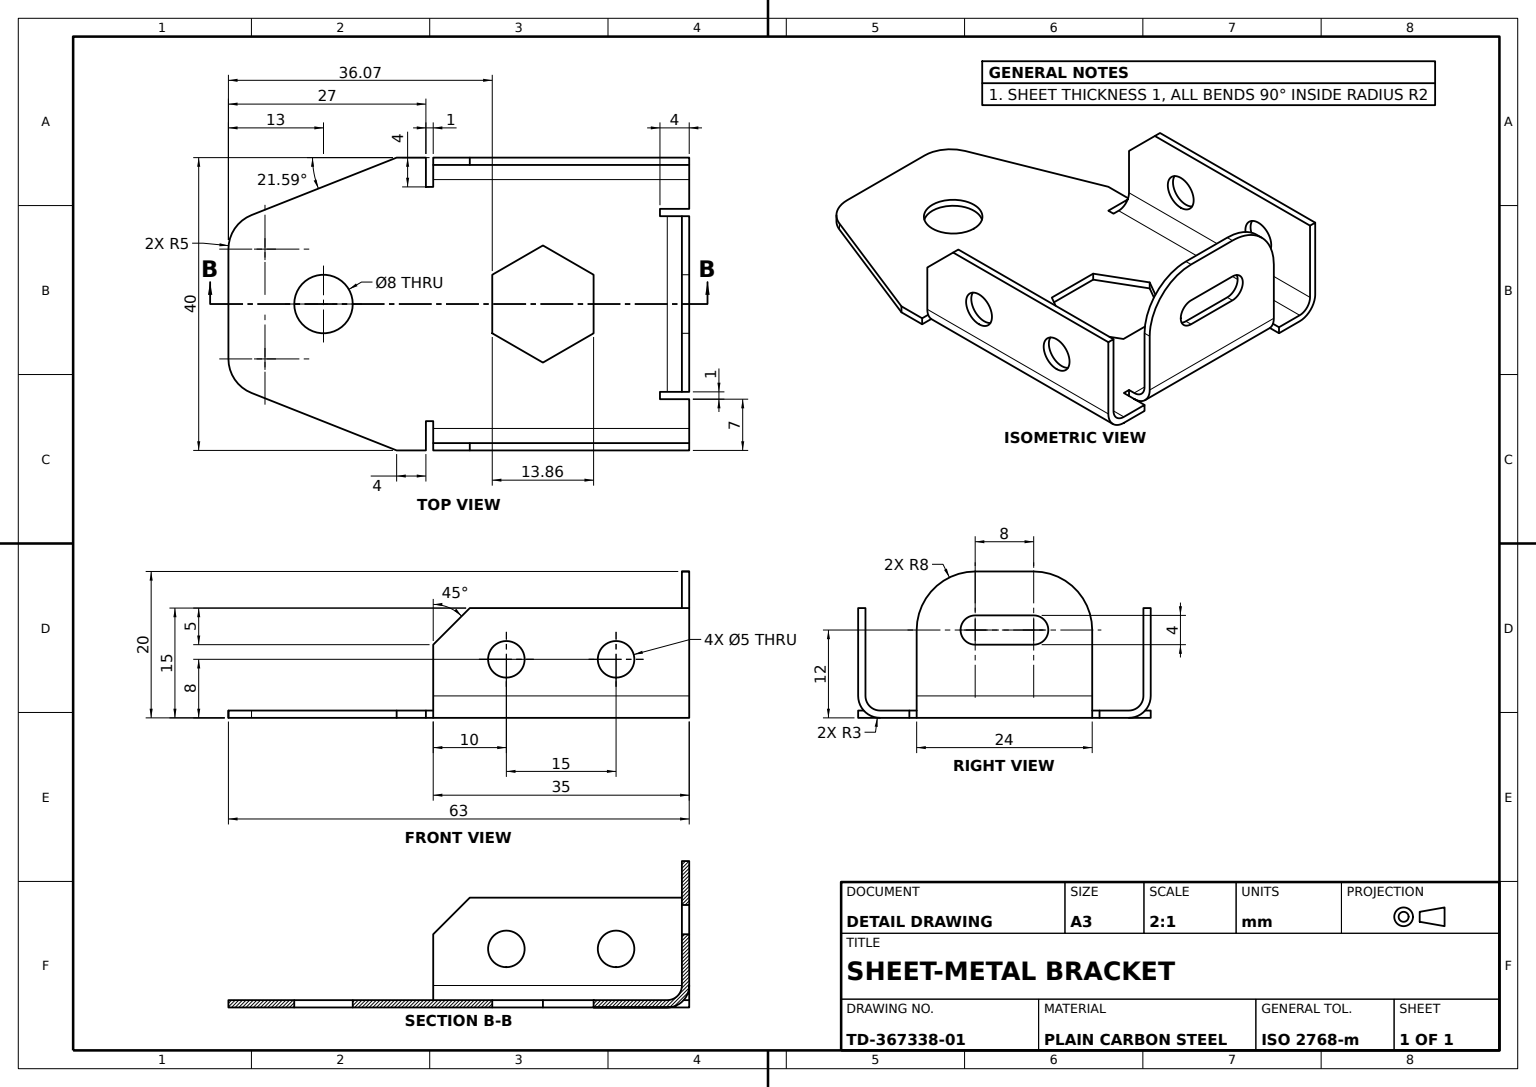
solid
v1 (20,9.5,-10)
v2 (20,4.5,-10)
e1 v1 v2 CIRCLE(AX(P(20,7,-10),D(1,0,0),D(0,1,0)),2.5)
e2 v2 v1 CIRCLE(AX(P(20,7,-10),D(1,0,0),D(0,1,0)),2.5)
v3 (20,2,-20)
v4 (20,2,15)
e3 v3 v4 LINE
v5 (20,14,-20)
e4 v3 v5 LINE
v6 (20,14,10)
e5 v5 v6 LINE
v7 (20,9,15)
e6 v6 v7 LINE
e7 v7 v4 LINE
v8 (20,9.5,5)
v9 (20,4.5,5)
e8 v8 v9 CIRCLE(AX(P(20,7,5),D(1,0,0),D(0,1,0)),2.5)
e9 v9 v8 CIRCLE(AX(P(20,7,5),D(1,0,0),D(0,1,0)),2.5)
face PLANE(AX(P(20,0,0),D(-1,0,0),D(0,-1,0))) rev [-e1 -e2] [-e3 e4 e5 e6 e7] [-e8 -e9]
v10 (-20,14,10)
v11 (-19,14,10)
e10 v10 v11 LINE
v12 (-20,9,15)
e11 v12 v10 LINE
v13 (-19,9,15)
e12 v13 v12 LINE
e13 v11 v13 LINE
face PLANE(AX(P(-20,14,10),D(0,-0.707106781,-0.707106781),D(1,0,0))) rev [-e10 -e11 -e12 -e13]
v14 (-4,0,-6.928203)
v15 (-8,0,0)
e14 v14 v15 LINE
v16 (-8,-1,0)
e15 v16 v15 LINE
v17 (-4,-1,-6.928203)
e16 v17 v16 LINE
e17 v17 v14 LINE
face PLANE(AX(P(-4,-1,-6.928203),D(-0.866025404,0,-0.5),D(-0.5,0,0.866025404))) rev [e14 -e15 -e16 e17]
v18 (-13,0,-16)
v19 (-12,0,-16)
e18 v18 v19 LINE
v20 (-12,-1,-16)
e19 v19 v20 LINE
v21 (-13,-1,-16)
e20 v20 v21 LINE
e21 v18 v21 LINE
face PLANE(AX(P(-13,0,-16),D(0,0,-1),D(0,1,0))) [e18 e19 e20 -e21]
v22 (-4,13,-20)
v23 (-4,13,-19)
e22 v22 v23 LINE
v24 (4,13,-20)
e23 v24 v22 LINE
v25 (4,13,-19)
e24 v24 v25 LINE
e25 v25 v23 LINE
face PLANE(AX(P(-4,13,-20),D(0,1,0),D(-1,0,0))) rev [-e22 -e23 e24 e25]
v26 (-17,0,-20)
v27 (-17,-1,-20)
e26 v26 v27 LINE
v28 (-20,2,-20)
e27 v27 v28 CIRCLE(AX(P(-17,2,-20),D(0,0,-1),D(1,0,0)),3)
v29 (-19,2,-20)
e28 v29 v28 LINE
e29 v26 v29 CIRCLE(AX(P(-17,2,-20),D(0,0,-1),D(1,0,0)),2)
face PLANE(AX(P(-17,2,-20),D(0,0,-1),D(-1,0,0))) [e26 e27 -e28 -e29]
v30 (17,-1,15)
e30 v30 v4 CIRCLE(AX(P(17,2,15),D(0,0,1),D(-1,0,0)),3)
v31 (17,-1,-20)
e31 v31 v30 LINE
e32 v3 v31 CIRCLE(AX(P(17,2,-20),D(0,0,-1),D(-1,0,0)),3)
face CYL(AX(P(17,2,-20),D(0,0,-1),D(1,0,0)),3) [-e30 -e31 -e32 e3]
v32 (-17,0,15)
e33 v32 v26 LINE
v33 (-19,2,15)
e34 v29 v33 LINE
e35 v33 v32 CIRCLE(AX(P(-17,2,15),D(0,0,1),D(1,0,0)),2)
face CYL(AX(P(-17,2,15),D(0,0,1),D(-1,0,0)),2) rev [e33 e29 e34 e35]
v34 (19,14,-20)
v35 (19,14,10)
e36 v34 v35 LINE
e37 v35 v6 LINE
e38 v5 v34 LINE
face PLANE(AX(P(20,14,15),D(0,-1,0),D(1,0,0))) rev [e36 e37 -e5 e38]
v36 (12,11,-19)
v37 (12,2,-19)
e39 v36 v37 LINE
v38 (12,2,-20)
e40 v37 v38 LINE
v39 (12,11,-20)
e41 v39 v38 LINE
e42 v39 v36 LINE
face PLANE(AX(P(12,0,-20),D(-1,0,0),D(0,0,1))) rev [e39 e40 -e41 e42]
v40 (0,-1,34)
v41 (0,0,34)
e43 v40 v41 LINE
v42 (0,0,26)
e44 v41 v42 CIRCLE(AX(P(0,0,30),D(0,1,0),D(0,0,1)),4)
v43 (0,-1,26)
e45 v43 v42 LINE
e46 v40 v43 CIRCLE(AX(P(0,-1,30),D(0,1,0),D(0,0,1)),4)
face CYL(AX(P(0,-1,30),D(0,1,0),D(0,0,1)),4) rev [e43 e44 -e45 -e46]
v44 (19,9.5,-10)
e47 v44 v1 LINE
v45 (19,4.5,-10)
e48 v45 v44 CIRCLE(AX(P(19,7,-10),D(1,0,0),D(0,1,0)),2.5)
e49 v45 v2 LINE
face CYL(AX(P(19,7,-10),D(1,0,0),D(0,1,0)),2.5) rev [-e47 -e48 e49 e2]
v46 (-20,2,15)
e50 v33 v46 LINE
v47 (-17,-1,15)
e51 v46 v47 CIRCLE(AX(P(-17,2,15),D(0,0,1),D(1,0,0)),3)
e52 v32 v47 LINE
face PLANE(AX(P(-17,2,15),D(0,0,-1),D(-1,0,0))) rev [-e35 e50 e51 -e52]
v48 (-4,9,-20)
e53 v22 v48 CIRCLE(AX(P(-4,11,-20),D(0,0,1),D(1,0,0)),2)
v49 (-4,9,-19)
e54 v23 v49 CIRCLE(AX(P(-4,11,-19),D(0,0,1),D(1,0,0)),2)
e55 v48 v49 LINE
face CYL(AX(P(-4,11,-20),D(0,0,1),D(1,0,0)),2) rev [-e53 e22 e54 -e55]
v50 (-19,4.5,5)
v51 (-20,4.5,5)
e56 v50 v51 LINE
v52 (-20,9.5,5)
e57 v52 v51 CIRCLE(AX(P(-20,7,5),D(1,0,0),D(0,1,0)),2.5)
v53 (-19,9.5,5)
e58 v53 v52 LINE
e59 v53 v50 CIRCLE(AX(P(-19,7,5),D(1,0,0),D(0,1,0)),2.5)
face CYL(AX(P(-19,7,5),D(-1,0,0),D(0,-1,0)),2.5) rev [e56 -e57 -e58 e59]
v54 (13,0,-20)
v55 (13,-1,-20)
e60 v54 v55 LINE
v56 (13,-1,-16)
e61 v55 v56 LINE
v57 (13,0,-16)
e62 v57 v56 LINE
e63 v57 v54 LINE
face PLANE(AX(P(13,0,-16),D(-1,0,0),D(0,0,1))) [e60 e61 -e62 e63]
v58 (19,9,15)
e64 v58 v35 LINE
e65 v7 v58 LINE
face PLANE(AX(P(20,9,15),D(0,-0.707106781,-0.707106781),D(-1,0,0))) rev [-e6 -e37 -e64 -e65]
v59 (19,9.5,5)
e66 v59 v8 LINE
v60 (19,4.5,5)
e67 v60 v59 CIRCLE(AX(P(19,7,5),D(1,0,0),D(0,1,0)),2.5)
e68 v60 v9 LINE
face CYL(AX(P(19,7,5),D(1,0,0),D(0,1,0)),2.5) rev [-e66 -e67 e68 e9]
v61 (6,11,-20)
v62 (6,11,-19)
e69 v61 v62 LINE
e70 v62 v25 CIRCLE(AX(P(4,11,-19),D(0,0,1),D(1,0,0)),2)
e71 v61 v24 CIRCLE(AX(P(4,11,-20),D(0,0,1),D(1,0,0)),2)
face CYL(AX(P(4,11,-20),D(0,0,1),D(1,0,0)),2) rev [e69 e70 -e24 -e71]
v63 (-20,-1,16)
v64 (-20,-1,20)
e72 v63 v64 LINE
v65 (-16,-1,16)
e73 v65 v63 LINE
v66 (-16,-1,15)
e74 v66 v65 LINE
e75 v47 v66 LINE
e76 v47 v27 LINE
v67 (-13,-1,-20)
e77 v67 v27 LINE
e78 v21 v67 LINE
v68 (-12,-1,-17)
e79 v68 v20 LINE
v69 (12,-1,-17)
e80 v68 v69 LINE
v70 (12,-1,-16)
e81 v70 v69 LINE
e82 v56 v70 LINE
e83 v31 v55 LINE
v71 (16,-1,15)
e84 v71 v30 LINE
v72 (16,-1,16)
e85 v72 v71 LINE
v73 (20,-1,16)
e86 v73 v72 LINE
v74 (20,-1,20)
e87 v74 v73 LINE
v75 (12.14923,-1,39.839743)
e88 v75 v74 LINE
v76 (7.5,-1,43)
e89 v76 v75 CIRCLE(AX(P(7.5,-1,38),D(0,1,0),D(0,0,1)),5)
v77 (-7.5,-1,43)
e90 v77 v76 LINE
v78 (-12.14923,-1,39.839743)
e91 v78 v77 CIRCLE(AX(P(-7.5,-1,38),D(0,1,0),D(0,0,1)),5)
e92 v64 v78 LINE
v79 (-4,-1,6.928203)
e93 v16 v79 LINE
v80 (4,-1,6.928203)
e94 v79 v80 LINE
v81 (8,-1,0)
e95 v80 v81 LINE
v82 (4,-1,-6.928203)
e96 v81 v82 LINE
e97 v82 v17 LINE
e98 v43 v40 CIRCLE(AX(P(0,-1,30),D(0,1,0),D(0,0,1)),4)
face PLANE(AX(P(-7.5,-1,38),D(0,1,0),D(0,0,1))) rev [-e72 -e73 -e74 -e75 e76 -e77 -e78 -e20 -e79 e80 -e81 -e82 -e61 -e83 e31 -e84 -e85 -e86 -e87 -e88 -e89 -e90 -e91 -e92] [e16 e93 e94 e95 e96 e97] [e46 e98]
v83 (-4,0,6.928203)
e99 v79 v83 LINE
v84 (4,0,6.928203)
e100 v83 v84 LINE
e101 v80 v84 LINE
face PLANE(AX(P(-4,-1,6.928203),D(0,0,1),D(1,0,0))) rev [e99 e100 -e101 -e94]
e102 v15 v83 LINE
face PLANE(AX(P(-8,-1,0),D(-0.866025404,0,0.5),D(0.5,0,0.866025404))) rev [e15 e102 -e99 -e93]
v85 (-20,0,20)
e103 v64 v85 LINE
v86 (-12.14923,0,39.839743)
e104 v78 v86 LINE
e105 v85 v86 LINE
face PLANE(AX(P(-20,-1,20),D(-0.929846099,0,0.36794868),D(0.36794868,0,0.929846099))) [-e103 e92 e104 -e105]
v87 (4,19,-20)
e106 v87 v39 CIRCLE(AX(P(4,11,-20),D(0,0,-1),D(0,-1,0)),8)
v88 (4,19,-19)
e107 v88 v87 LINE
e108 v36 v88 CIRCLE(AX(P(4,11,-19),D(0,0,1),D(0,-1,0)),8)
face CYL(AX(P(4,11,-20),D(0,0,1),D(0,-1,0)),8) [-e106 -e107 -e108 -e42]
v89 (-16,0,16)
e109 v89 v65 LINE
v90 (-20,0,16)
e110 v90 v63 LINE
e111 v90 v89 LINE
face PLANE(AX(P(-20,0,16),D(0,0,-1),D(0,1,0))) [e109 e73 -e110 e111]
v91 (-12,2,-20)
v92 (-12,11,-20)
e112 v91 v92 LINE
v93 (-12,2,-19)
e113 v93 v91 LINE
v94 (-12,11,-19)
e114 v93 v94 LINE
e115 v94 v92 LINE
face PLANE(AX(P(-12,19,-20),D(1,0,0),D(0,0,-1))) rev [-e112 -e113 e114 e115]
v95 (4,9,-19)
e116 v95 v62 CIRCLE(AX(P(4,11,-19),D(0,0,1),D(1,0,0)),2)
v96 (4,9,-20)
e117 v96 v61 CIRCLE(AX(P(4,11,-20),D(0,0,1),D(1,0,0)),2)
e118 v96 v95 LINE
face CYL(AX(P(4,11,-20),D(0,0,1),D(1,0,0)),2) rev [e116 -e69 -e117 e118]
e119 v51 v52 CIRCLE(AX(P(-20,7,5),D(1,0,0),D(0,1,0)),2.5)
e120 v50 v53 CIRCLE(AX(P(-19,7,5),D(1,0,0),D(0,1,0)),2.5)
face CYL(AX(P(-19,7,5),D(-1,0,0),D(0,-1,0)),2.5) rev [e58 -e119 -e56 e120]
e121 v42 v41 CIRCLE(AX(P(0,0,30),D(0,1,0),D(0,0,1)),4)
v97 (-7.5,0,43)
e122 v86 v97 CIRCLE(AX(P(-7.5,0,38),D(0,1,0),D(0,0,1)),5)
v98 (7.5,0,43)
e123 v97 v98 LINE
v99 (12.14923,0,39.839743)
e124 v98 v99 CIRCLE(AX(P(7.5,0,38),D(0,1,0),D(0,0,1)),5)
v100 (20,0,20)
e125 v99 v100 LINE
v101 (20,0,16)
e126 v100 v101 LINE
v102 (16,0,16)
e127 v102 v101 LINE
v103 (16,0,15)
e128 v103 v102 LINE
v104 (17,0,15)
e129 v104 v103 LINE
v105 (17,0,-20)
e130 v105 v104 LINE
e131 v105 v54 LINE
v106 (12,0,-16)
e132 v106 v57 LINE
v107 (12,0,-17)
e133 v107 v106 LINE
v108 (-12,0,-17)
e134 v108 v107 LINE
e135 v19 v108 LINE
v109 (-13,0,-20)
e136 v109 v18 LINE
e137 v109 v26 LINE
v110 (-16,0,15)
e138 v110 v32 LINE
e139 v89 v110 LINE
e140 v90 v85 LINE
v111 (4,0,-6.928203)
e141 v111 v14 LINE
v112 (8,0,0)
e142 v112 v111 LINE
e143 v84 v112 LINE
face PLANE(AX(P(-7.5,0,38),D(0,1,0),D(0,0,1))) [-e121 -e44] [e122 e123 e124 e125 e126 -e127 -e128 -e129 -e130 e131 -e63 -e132 -e133 -e134 -e135 -e18 -e136 e137 -e33 -e138 -e139 -e111 e140 e105] [-e141 -e142 -e143 -e100 -e102 -e14]
e144 v49 v95 LINE
e145 v48 v96 LINE
face PLANE(AX(P(-4,9,-20),D(0,-1,0),D(1,0,0))) rev [e55 e144 -e118 -e145]
e146 v109 v67 LINE
face PLANE(AX(P(-20,-1,-20),D(0,0,-1),D(-1,0,0))) [e146 e77 -e26 -e137]
v113 (19,2,-20)
e147 v113 v3 LINE
e148 v113 v34 LINE
face PLANE(AX(P(20,14,-20),D(0,0,1),D(1,0,0))) rev [-e38 -e4 -e147 e148]
e149 v103 v71 LINE
e150 v104 v30 LINE
face PLANE(AX(P(17,0,15),D(0,0,1),D(0,-1,0))) [e129 e149 e84 -e150]
e151 v82 v111 LINE
face PLANE(AX(P(4,-1,-6.928203),D(0,0,-1),D(-1,0,0))) rev [e141 -e17 -e97 e151]
e152 v113 v105 CIRCLE(AX(P(17,2,-20),D(0,0,-1),D(-1,0,0)),2)
v114 (19,2,15)
e153 v104 v114 CIRCLE(AX(P(17,2,15),D(0,0,1),D(-1,0,0)),2)
e154 v114 v113 LINE
face CYL(AX(P(17,2,-20),D(0,0,-1),D(1,0,0)),2) rev [e152 e130 e153 e154]
v115 (-20,14,-20)
e155 v115 v10 LINE
e156 v28 v115 LINE
e157 v46 v28 LINE
e158 v12 v46 LINE
v116 (-20,9.5,-10)
v117 (-20,4.5,-10)
e159 v116 v117 CIRCLE(AX(P(-20,7,-10),D(1,0,0),D(0,1,0)),2.5)
e160 v117 v116 CIRCLE(AX(P(-20,7,-10),D(1,0,0),D(0,1,0)),2.5)
face PLANE(AX(P(-20,0,0),D(1,0,0),D(0,-1,0))) rev [e57 e119] [e11 -e155 -e156 -e157 -e158] [e159 e160]
v118 (-19,9.5,-10)
e161 v118 v116 LINE
v119 (-19,4.5,-10)
e162 v119 v117 LINE
e163 v119 v118 CIRCLE(AX(P(-19,7,-10),D(1,0,0),D(0,1,0)),2.5)
face CYL(AX(P(-19,7,-10),D(-1,0,0),D(0,-1,0)),2.5) rev [e161 -e160 -e162 e163]
e164 v105 v31 LINE
face PLANE(AX(P(17,2,-20),D(0,0,1),D(1,0,0))) rev [e147 e32 -e164 -e152]
e165 v77 v97 LINE
e166 v76 v98 LINE
face PLANE(AX(P(-7.5,-1,43),D(0,0,1),D(1,0,0))) [-e165 e90 e166 -e123]
v120 (-19,14,-20)
e167 v29 v120 LINE
e168 v120 v11 LINE
e169 v13 v33 LINE
e170 v118 v119 CIRCLE(AX(P(-19,7,-10),D(1,0,0),D(0,1,0)),2.5)
face PLANE(AX(P(-19,0,0),D(1,0,0),D(0,-1,0))) [-e34 e167 e168 e13 e169] [-e170 -e163] [-e59 -e120]
e171 v110 v66 LINE
face PLANE(AX(P(-16,0,16),D(-1,0,0),D(0,0,1))) [-e109 e139 e171 e74]
e172 v107 v37 CIRCLE(AX(P(12,2,-17),D(1,0,0),D(0,0,1)),2)
e173 v107 v69 LINE
e174 v69 v38 CIRCLE(AX(P(12,2,-17),D(1,0,0),D(0,0,1)),3)
face PLANE(AX(P(12,2,-17),D(1,0,0),D(0,0,-1))) [-e40 -e172 e173 e174]
e175 v91 v38 LINE
v121 (-4,19,-20)
e176 v92 v121 CIRCLE(AX(P(-4,11,-20),D(0,0,-1),D(0,-1,0)),8)
e177 v121 v87 LINE
face PLANE(AX(P(0,0,-20),D(0,0,1),D(0,-1,0))) rev [e117 e71 e23 e53 e145] [e106 e41 -e175 e112 e176 e177]
v122 (-4,19,-19)
e178 v121 v122 LINE
e179 v122 v88 LINE
face PLANE(AX(P(12,19,-20),D(0,-1,0),D(0,0,-1))) rev [-e177 e178 e179 e107]
e180 v102 v72 LINE
face PLANE(AX(P(16,0,15),D(1,0,0),D(0,0,-1))) [e180 e85 -e149 e128]
face PLANE(AX(P(-20,-1,20),D(-1,0,0),D(0,0,1))) [e72 e103 -e140 e110]
e181 v106 v70 LINE
face PLANE(AX(P(12,0,-17),D(1,0,0),D(0,0,-1))) [-e173 e133 e181 e81]
e182 v74 v100 LINE
e183 v101 v73 LINE
face PLANE(AX(P(20,-1,20),D(1,0,0),D(0,0,-1))) [-e126 -e182 e87 -e183]
e184 v108 v68 LINE
face PLANE(AX(P(-12,0,-16),D(-1,0,0),D(0,0,1))) [e79 -e19 e135 e184]
e185 v81 v112 LINE
face PLANE(AX(P(4,-1,6.928203),D(0.866025404,0,0.5),D(0.5,0,-0.866025404))) rev [-e95 e101 e143 -e185]
face CYL(AX(P(-17,2,15),D(0,0,1),D(-1,0,0)),3) [e157 -e27 -e76 -e51]
e186 v91 v68 CIRCLE(AX(P(-12,2,-17),D(-1,0,0),D(0,0,1)),3)
face CYL(AX(P(-12,2,-17),D(-1,0,0),D(0,0,-1)),3) [e175 -e174 -e80 -e186]
e187 v44 v45 CIRCLE(AX(P(19,7,-10),D(1,0,0),D(0,1,0)),2.5)
e188 v58 v114 LINE
e189 v59 v60 CIRCLE(AX(P(19,7,5),D(1,0,0),D(0,1,0)),2.5)
face PLANE(AX(P(19,0,0),D(-1,0,0),D(0,-1,0))) [e48 e187] [-e188 e64 -e36 -e148 -e154] [e67 e189]
face PLANE(AX(P(12,0,-16),D(0,0,-1),D(0,1,0))) [e82 -e181 e132 e62]
e190 v93 v108 CIRCLE(AX(P(-12,2,-17),D(-1,0,0),D(0,0,1)),2)
face PLANE(AX(P(-12,2,-17),D(1,0,0),D(0,0,-1))) rev [e186 -e184 -e190 e113]
e191 v122 v94 CIRCLE(AX(P(-4,11,-19),D(0,0,1),D(0,-1,0)),8)
face CYL(AX(P(-4,11,-20),D(0,0,1),D(0,-1,0)),8) [-e115 -e191 -e178 -e176]
e192 v37 v93 LINE
face CYL(AX(P(-12,2,-17),D(-1,0,0),D(0,0,-1)),2) rev [e192 e190 e134 e172]
e193 v115 v120 LINE
face PLANE(AX(P(-20,14,-20),D(0,0,-1),D(-1,0,0))) [e193 -e167 e28 e156]
face CYL(AX(P(19,7,-10),D(1,0,0),D(0,1,0)),2.5) rev [e1 -e49 -e187 e47]
face CYL(AX(P(0,-1,30),D(0,1,0),D(0,0,1)),4) rev [e121 -e43 -e98 e45]
face PLANE(AX(P(-16,0,15),D(0,0,1),D(0,-1,0))) [e75 -e171 e138 e52]
e194 v75 v99 LINE
face CYL(AX(P(7.5,-1,38),D(0,1,0),D(0,0,1)),5) [-e166 e89 e194 -e124]
face PLANE(AX(P(-20,14,15),D(0,1,0),D(-1,0,0))) [-e193 e155 e10 -e168]
face PLANE(AX(P(16,0,16),D(0,0,-1),D(0,1,0))) [e183 e86 -e180 e127]
e195 v114 v4 LINE
face PLANE(AX(P(20,0,15),D(0,0,-1),D(-1,0,0))) rev [e195 -e7 e65 e188]
face PLANE(AX(P(-20,-1,-20),D(0,0,-1),D(-1,0,0))) [-e131 e164 e83 -e60]
face PLANE(AX(P(0,0,-19),D(0,0,1),D(0,-1,0))) [-e114 -e192 -e39 e108 -e179 e191] [-e54 -e25 -e70 -e116 -e144]
face PLANE(AX(P(12.14923,-1,39.839743),D(0.929846099,0,0.36794868),D(0.36794868,0,-0.929846099))) [e182 -e125 -e194 e88]
face PLANE(AX(P(8,-1,0),D(0.866025404,0,-0.5),D(-0.5,0,-0.866025404))) rev [e142 -e151 -e96 e185]
face PLANE(AX(P(-20,0,15),D(0,0,1),D(1,0,0))) [-e50 -e169 e12 e158]
face CYL(AX(P(19,7,5),D(1,0,0),D(0,1,0)),2.5) rev [-e68 -e189 e66 e8]
face CYL(AX(P(-19,7,-10),D(-1,0,0),D(0,-1,0)),2.5) rev [e170 e162 -e159 -e161]
face CYL(AX(P(-7.5,-1,38),D(0,1,0),D(0,0,1)),5) [e91 e165 -e122 -e104]
face PLANE(AX(P(17,2,15),D(0,0,1),D(1,0,0))) [e150 e30 -e195 -e153]
face PLANE(AX(P(-13,0,-20),D(1,0,0),D(0,0,-1))) [-e146 e136 e21 e78]
